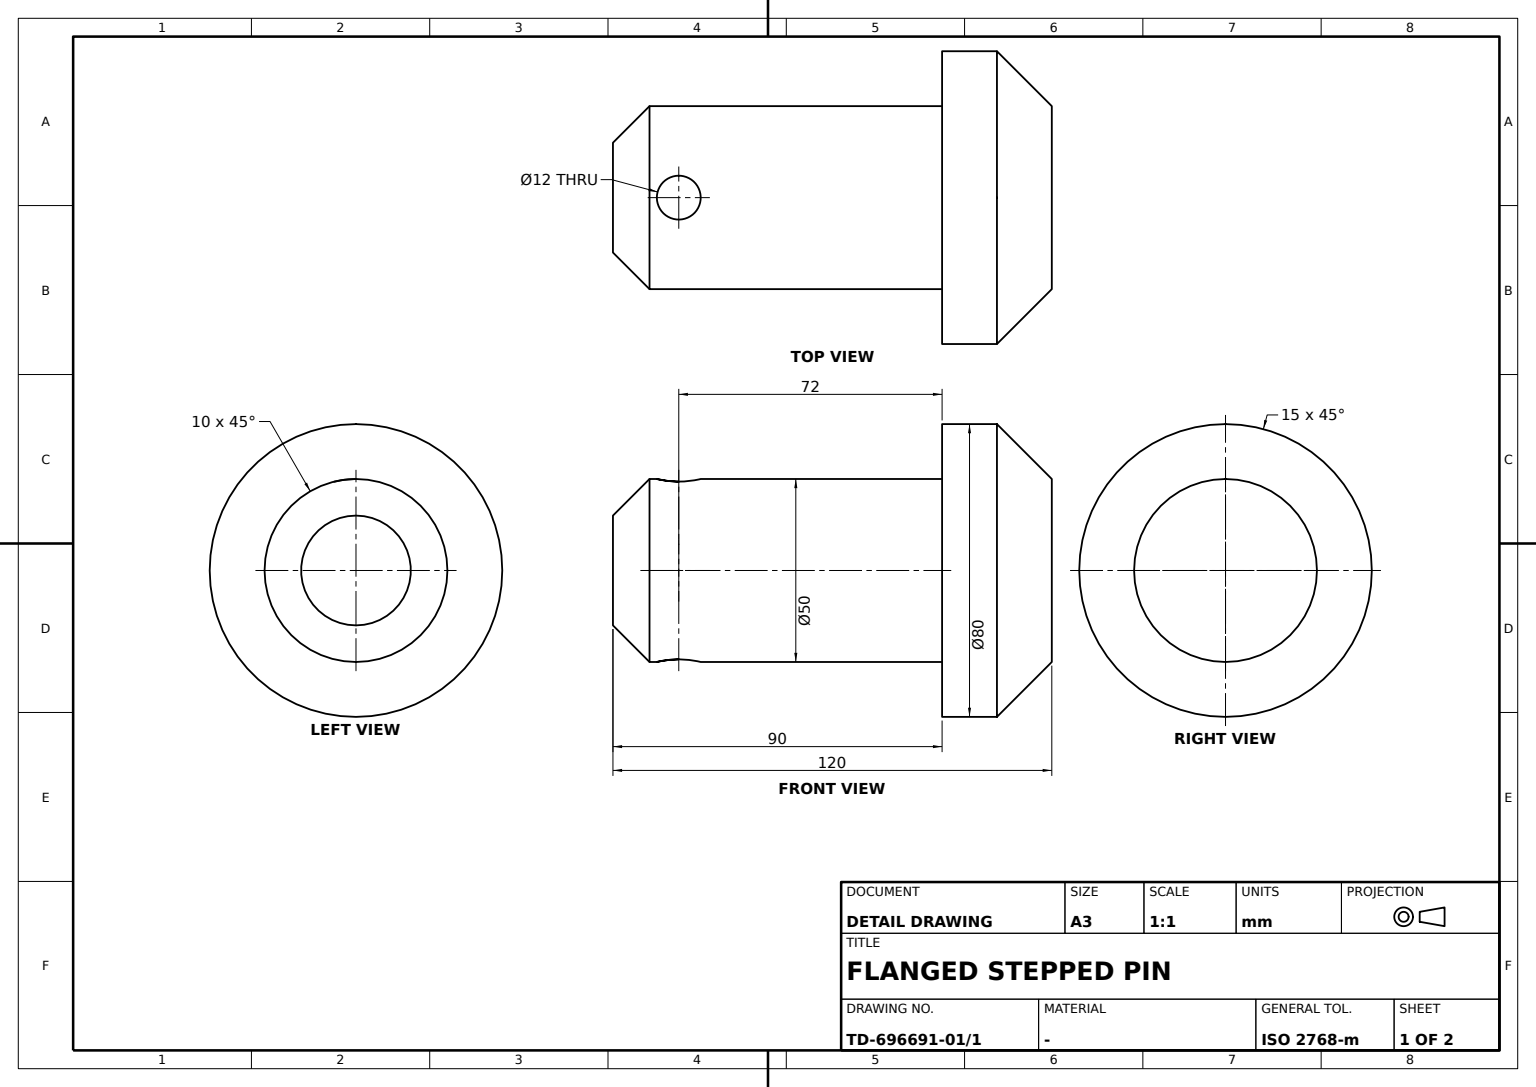
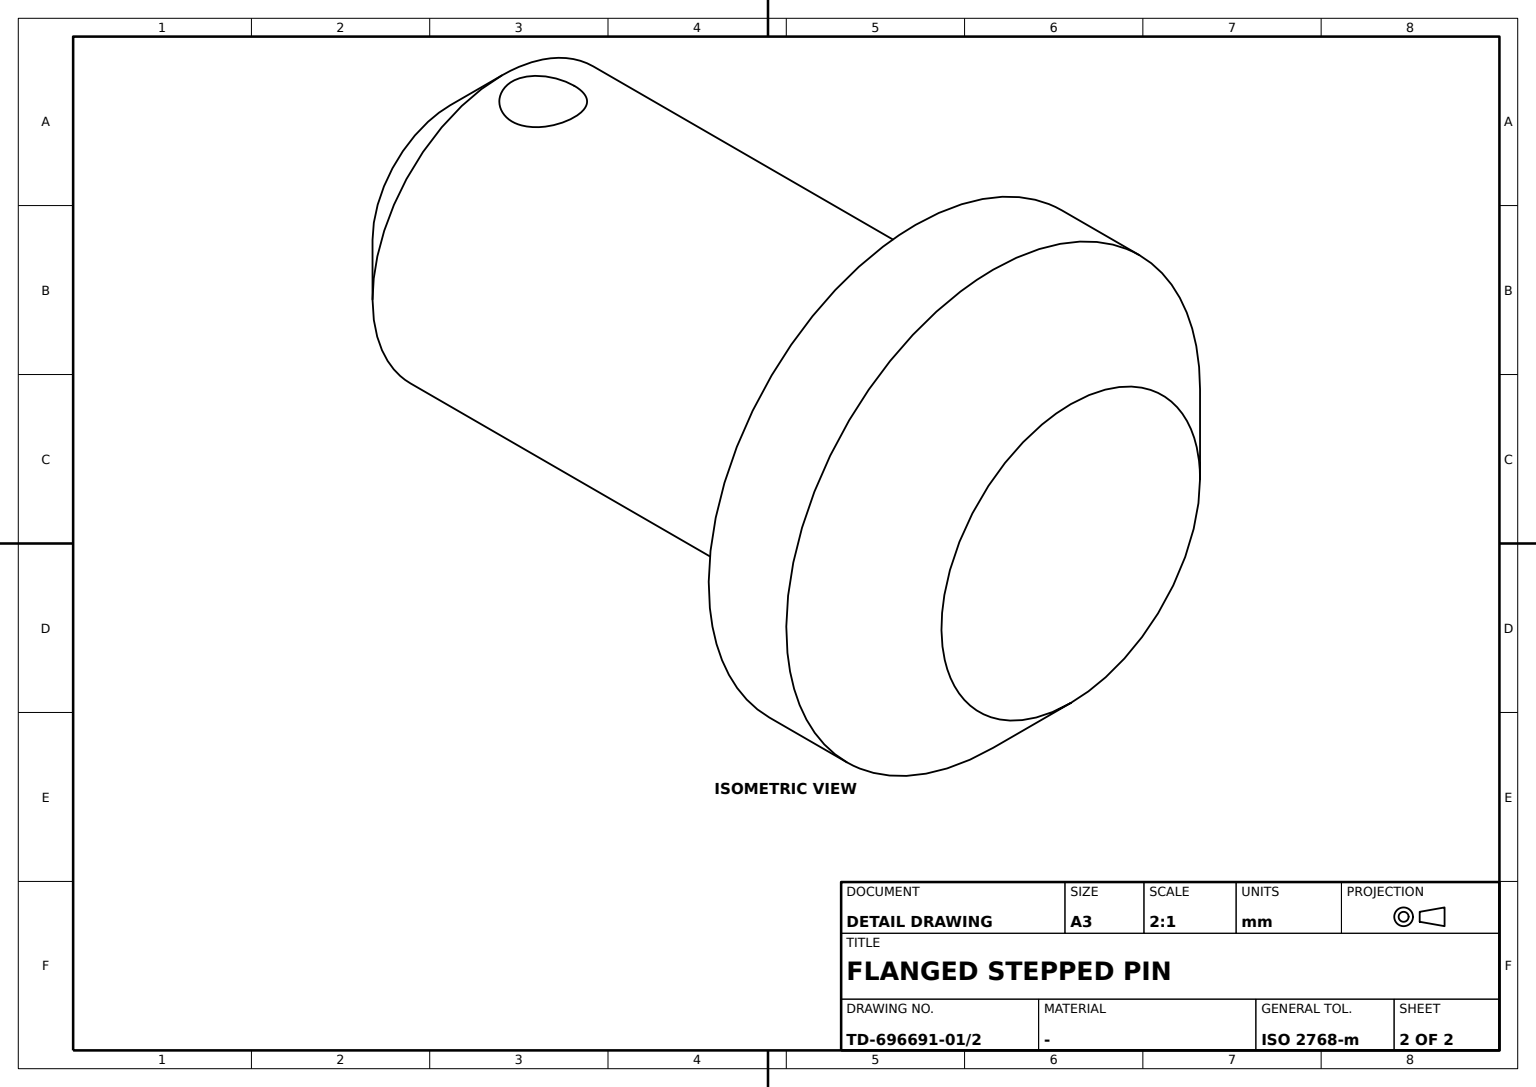
ISO-10303-21;
HEADER;
FILE_DESCRIPTION((''),'2;1');
FILE_NAME('','',(''),(''),'','','');
FILE_SCHEMA(('AUTOMOTIVE_DESIGN'));
ENDSEC;
DATA;
#1=APPLICATION_CONTEXT('');
#2=PRODUCT_CONTEXT('',#1,'mechanical');
#3=PRODUCT('','','',(#2));
#4=PRODUCT_DEFINITION_FORMATION('','',#3);
#5=PRODUCT_DEFINITION_CONTEXT('',#1,'design');
#6=PRODUCT_DEFINITION('','',#4,#5);
#7=PRODUCT_DEFINITION_SHAPE('','',#6);
#8=(LENGTH_UNIT()NAMED_UNIT(*)SI_UNIT(.MILLI.,.METRE.));
#9=(NAMED_UNIT(*)PLANE_ANGLE_UNIT()SI_UNIT($,.RADIAN.));
#10=(NAMED_UNIT(*)SI_UNIT($,.STERADIAN.)SOLID_ANGLE_UNIT());
#11=UNCERTAINTY_MEASURE_WITH_UNIT(LENGTH_MEASURE(0.005),#8,'distance_accuracy_value','');
#12=(GEOMETRIC_REPRESENTATION_CONTEXT(3)GLOBAL_UNCERTAINTY_ASSIGNED_CONTEXT((#11))GLOBAL_UNIT_ASSIGNED_CONTEXT((#8,#9,#10))REPRESENTATION_CONTEXT('',''));
#13=CARTESIAN_POINT('',(-102.,6.,24.269322));
#14=VERTEX_POINT('',#13);
#15=CARTESIAN_POINT('',(-97.295047,4.700662,24.640652));
#16=CARTESIAN_POINT('',(-102.000852,6.649955,24.083785));
#17=CARTESIAN_POINT('',(-106.701546,4.699519,24.640141));
#18=CARTESIAN_POINT('',(-108.648362,0.008261,25.179796));
#19=CARTESIAN_POINT('',(-106.704992,-4.700557,24.640673));
#20=CARTESIAN_POINT('',(-101.999427,-6.649955,24.083785));
#21=CARTESIAN_POINT('',(-97.298493,-4.699622,24.64012));
#22=CARTESIAN_POINT('',(-95.351619,-0.008261,25.179806));
#23=B_SPLINE_CURVE_WITH_KNOTS('',3,(#15,#16,#17,#18,#19,#20,#21,#22,#15,#16,#17),.UNSPECIFIED.,.T.,.F.,(1,1,1,1,1,1,1,1,1,1,1,1,1,1,1),(-0.014116296,-0.009410864,-0.004705432,0.,0.004705432,0.009410864,0.014116296,0.018821728,0.023527161,0.028232593,0.032938025,0.037643457,0.042348889,0.047054321,0.051759753),.UNSPECIFIED.);
#24=EDGE_CURVE('',#14,#14,#23,.T.);
#25=ORIENTED_EDGE('',*,*,#24,.T.);
#26=EDGE_LOOP('',(#25));
#27=FACE_BOUND('',#26,.T.);
#28=CARTESIAN_POINT('',(-102.,-6.,-24.269322));
#29=VERTEX_POINT('',#28);
#30=CARTESIAN_POINT('',(-106.704953,-4.700662,-24.640652));
#31=CARTESIAN_POINT('',(-101.999148,-6.649955,-24.083785));
#32=CARTESIAN_POINT('',(-97.298454,-4.699519,-24.640141));
#33=CARTESIAN_POINT('',(-95.351638,-0.008261,-25.179796));
#34=CARTESIAN_POINT('',(-97.295008,4.700557,-24.640673));
#35=CARTESIAN_POINT('',(-102.000573,6.649955,-24.083785));
#36=CARTESIAN_POINT('',(-106.701507,4.699622,-24.64012));
#37=CARTESIAN_POINT('',(-108.648381,0.008261,-25.179806));
#38=B_SPLINE_CURVE_WITH_KNOTS('',3,(#30,#31,#32,#33,#34,#35,#36,#37,#30,#31,#32),.UNSPECIFIED.,.T.,.F.,(1,1,1,1,1,1,1,1,1,1,1,1,1,1,1),(-0.014116296,-0.009410864,-0.004705432,0.,0.004705432,0.009410864,0.014116296,0.018821728,0.023527161,0.028232593,0.032938025,0.037643457,0.042348889,0.047054321,0.051759753),.UNSPECIFIED.);
#39=EDGE_CURVE('',#29,#29,#38,.F.);
#40=ORIENTED_EDGE('',*,*,#39,.T.);
#41=EDGE_LOOP('',(#40));
#42=FACE_BOUND('',#41,.T.);
#43=CARTESIAN_POINT('',(-102.,0.,0.));
#44=DIRECTION('',(0.,0.,1.));
#45=DIRECTION('',(0.,1.,0.));
#46=AXIS2_PLACEMENT_3D('',#43,#44,#45);
#47=CYLINDRICAL_SURFACE('',#46,6.);
#48=ADVANCED_FACE('',(#27,#42),#47,.F.);
#49=CARTESIAN_POINT('',(0.,0.,25.));
#50=VERTEX_POINT('',#49);
#51=CARTESIAN_POINT('',(0.,0.,0.));
#52=DIRECTION('',(-1.,0.,0.));
#53=AXIS2_PLACEMENT_3D('',#51,#52,#44);
#54=CIRCLE('',#53,25.);
#55=EDGE_CURVE('',#50,#50,#54,.T.);
#56=ORIENTED_EDGE('',*,*,#55,.T.);
#57=EDGE_LOOP('',(#56));
#58=FACE_BOUND('',#57,.T.);
#59=CARTESIAN_POINT('',(-15.,0.,40.));
#60=VERTEX_POINT('',#59);
#61=CARTESIAN_POINT('',(-15.,0.,0.));
#62=AXIS2_PLACEMENT_3D('',#61,#52,#44);
#63=CIRCLE('',#62,40.);
#64=EDGE_CURVE('',#60,#60,#63,.T.);
#65=ORIENTED_EDGE('',*,*,#64,.F.);
#66=EDGE_LOOP('',(#65));
#67=FACE_BOUND('',#66,.T.);
#68=CARTESIAN_POINT('',(25.,0.,0.));
#69=DIRECTION('',(0.,-1.,0.));
#70=AXIS2_PLACEMENT_3D('',#68,#52,#69);
#71=CONICAL_SURFACE('',#70,0.,0.785398163);
#72=ADVANCED_FACE('',(#58,#67),#71,.T.);
#73=ORIENTED_EDGE('',*,*,#55,.F.);
#74=EDGE_LOOP('',(#73));
#75=FACE_BOUND('',#74,.T.);
#76=AXIS2_PLACEMENT_3D('',#51,#52,#69);
#77=PLANE('',#76);
#78=ADVANCED_FACE('',(#75),#77,.F.);
#79=ORIENTED_EDGE('',*,*,#64,.T.);
#80=EDGE_LOOP('',(#79));
#81=FACE_BOUND('',#80,.T.);
#82=CARTESIAN_POINT('',(-30.,0.,40.));
#83=VERTEX_POINT('',#82);
#84=CARTESIAN_POINT('',(-30.,0.,0.));
#85=AXIS2_PLACEMENT_3D('',#84,#52,#44);
#86=CIRCLE('',#85,40.);
#87=EDGE_CURVE('',#83,#83,#86,.T.);
#88=ORIENTED_EDGE('',*,*,#87,.F.);
#89=EDGE_LOOP('',(#88));
#90=FACE_BOUND('',#89,.T.);
#91=AXIS2_PLACEMENT_3D('',#61,#52,#69);
#92=CYLINDRICAL_SURFACE('',#91,40.);
#93=ADVANCED_FACE('',(#81,#90),#92,.T.);
#94=CARTESIAN_POINT('',(-110.,0.,-25.));
#95=VERTEX_POINT('',#94);
#96=CARTESIAN_POINT('',(-110.,0.,0.));
#97=DIRECTION('',(1.,0.,0.));
#98=DIRECTION('',(0.,0.,-1.));
#99=AXIS2_PLACEMENT_3D('',#96,#97,#98);
#100=CIRCLE('',#99,25.);
#101=EDGE_CURVE('',#95,#95,#100,.F.);
#102=ORIENTED_EDGE('',*,*,#101,.F.);
#103=EDGE_LOOP('',(#102));
#104=FACE_BOUND('',#103,.T.);
#105=ORIENTED_EDGE('',*,*,#39,.F.);
#106=EDGE_LOOP('',(#105));
#107=FACE_BOUND('',#106,.T.);
#108=ORIENTED_EDGE('',*,*,#24,.F.);
#109=EDGE_LOOP('',(#108));
#110=FACE_BOUND('',#109,.T.);
#111=CARTESIAN_POINT('',(-30.,0.,25.));
#112=VERTEX_POINT('',#111);
#113=CIRCLE('',#85,25.);
#114=EDGE_CURVE('',#112,#112,#113,.T.);
#115=ORIENTED_EDGE('',*,*,#114,.T.);
#116=EDGE_LOOP('',(#115));
#117=FACE_BOUND('',#116,.T.);
#118=CARTESIAN_POINT('',(-75.,0.,0.));
#119=AXIS2_PLACEMENT_3D('',#118,#52,#69);
#120=CYLINDRICAL_SURFACE('',#119,25.);
#121=ADVANCED_FACE('',(#104,#107,#110,#117),#120,.T.);
#122=CARTESIAN_POINT('',(-120.,0.,15.));
#123=VERTEX_POINT('',#122);
#124=CARTESIAN_POINT('',(-120.,0.,0.));
#125=AXIS2_PLACEMENT_3D('',#124,#52,#44);
#126=CIRCLE('',#125,15.);
#127=EDGE_CURVE('',#123,#123,#126,.T.);
#128=ORIENTED_EDGE('',*,*,#127,.F.);
#129=EDGE_LOOP('',(#128));
#130=FACE_BOUND('',#129,.T.);
#131=ORIENTED_EDGE('',*,*,#101,.T.);
#132=EDGE_LOOP('',(#131));
#133=FACE_BOUND('',#132,.T.);
#134=CARTESIAN_POINT('',(-135.,0.,0.));
#135=AXIS2_PLACEMENT_3D('',#134,#97,#45);
#136=CONICAL_SURFACE('',#135,0.,0.785398163);
#137=ADVANCED_FACE('',(#130,#133),#136,.T.);
#138=ORIENTED_EDGE('',*,*,#127,.T.);
#139=EDGE_LOOP('',(#138));
#140=FACE_BOUND('',#139,.T.);
#141=AXIS2_PLACEMENT_3D('',#124,#52,#69);
#142=PLANE('',#141);
#143=ADVANCED_FACE('',(#140),#142,.T.);
#144=ORIENTED_EDGE('',*,*,#87,.T.);
#145=EDGE_LOOP('',(#144));
#146=FACE_BOUND('',#145,.T.);
#147=ORIENTED_EDGE('',*,*,#114,.F.);
#148=EDGE_LOOP('',(#147));
#149=FACE_BOUND('',#148,.T.);
#150=AXIS2_PLACEMENT_3D('',#84,#52,#69);
#151=PLANE('',#150);
#152=ADVANCED_FACE('',(#146,#149),#151,.T.);
#153=CLOSED_SHELL('',(#48,#72,#78,#93,#121,#137,#143,#152));
#154=MANIFOLD_SOLID_BREP('',#153);
#155=ADVANCED_BREP_SHAPE_REPRESENTATION('',(#154),#12);
#156=SHAPE_DEFINITION_REPRESENTATION(#7,#155);
ENDSEC;
END-ISO-10303-21;
